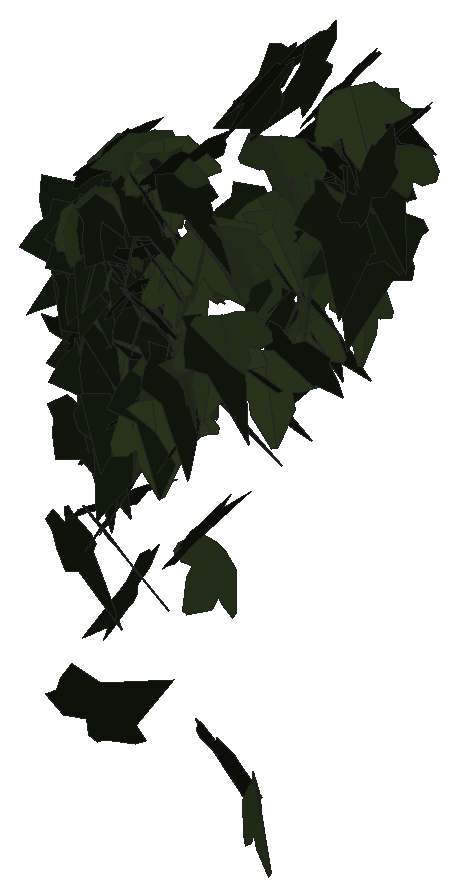
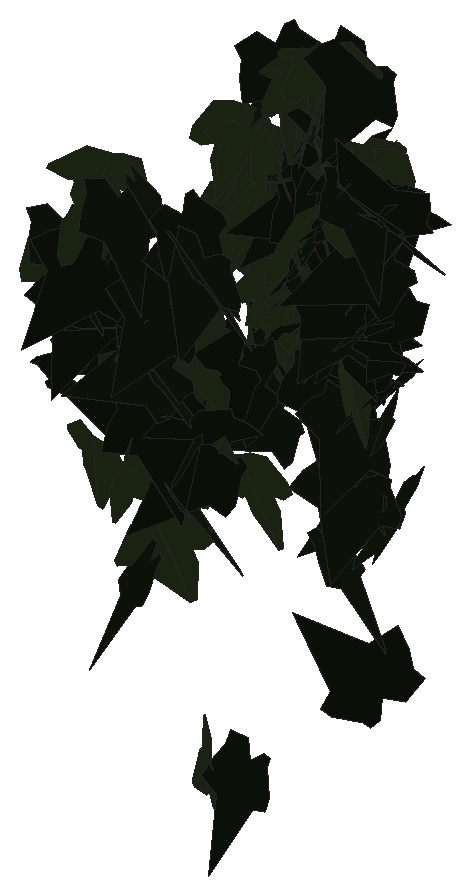
# SketchUp Ruby script. Lengths in inches.
U = 1.inch
M = Sketchup.active_model
def pt(a) = Geom::Point3d.new(a.map { |v| v * U })
def face(e, loops, mat)
  f = e.add_face(loops[0].map { |a| pt(a) })
  loops[1..].each { |l| e.add_face(l.map { |a| pt(a) }).erase! }
  f.material = f.back_material = mat if mat
  f
end
# faces: each face lists its corners as indices into pts; further lists are holes
def faces(e, pts, list, mat = nil) = list.each { |f| face(e, (f[0].is_a?(Array) ? f : [f]).map { |l| l.map { |i| pts[i] } }, mat) }
# xy, xz, yz: faces in a plane at the given z, y or x. An outline is a flat list of corners, or four numbers for a rectangle; further outlines are holes
def ring(l) = l.size == 4 ? [[l[0], l[1]], [l[2], l[1]], [l[2], l[3]], [l[0], l[3]]] : l.each_slice(2).to_a
def flat(e, list, mat, &to3) = list.each { |f| face(e, (f[0].is_a?(Array) ? f : [f]).map { |l| ring(l).map { |u, v| to3.(u, v) } }, mat) }
def xy(e, z, list, mat = nil) = flat(e, list, mat) { |x, y| [x, y, z] }
def xz(e, y, list, mat = nil) = flat(e, list, mat) { |x, z| [x, y, z] }
def yz(e, x, list, mat = nil) = flat(e, list, mat) { |y, z| [x, y, z] }
def lines(e, pts, list) = list.each { |a, b| e.add_line(pt(pts[a]), pt(pts[b])) }
# prism: a flat outline (further loops are holes) pulled along v
def prism(e, loops, v, mat = nil)
  f = face(e, loops, mat); d = Geom::Vector3d.new(v.map { |x| x * U })
  f.pushpull(f.normal.samedirection?(d) ? d.length : -d.length)
end
def box(e, o, s, mat = nil) = prism(e, [[o, [o[0] + s[0], o[1], o[2]], [o[0] + s[0], o[1] + s[1], o[2]], [o[0], o[1] + s[1], o[2]]]], [0, 0, s[2]], mat)
def at(x, y, z, deg = 0) = Geom::Transformation.translation(pt([x, y, z])) * Geom::Transformation.rotation(ORIGIN, Z_AXIS, deg.degrees)
def axes(o, x, y, z) = Geom::Transformation.new([*x, 0, *y, 0, *z, 0, *pt(o).to_a, 1])
def part(name) = M.definitions.add(name)
# library, detail: a bought-in or finely detailed component or shape, given as its bounding box
def library(name, o, s) = part(name).tap { |d| box(d.entities, o, s) }
def detail(e, o, s) = box(e.add_group.entities, o, s)
def put(e, d, t, mat = nil) = e.add_instance(d, t).tap { |i| i.material = mat if mat }
def group(e, t, mat = nil) = e.add_group.tap { |g| g.transformation = t; g.material = mat if mat }.entities
root = M.entities
M.materials.add("efeu1").color = [18, 25, 13]
M.materials.add("efeu2").color = [43, 57, 29]
c1 = part("ivyleaf_10")
p = [[0,0.5,-0.03],[-0.0625,2.02,-0.43],[-0.19,2.01,-0.46],[-0.54,1.05,-0.29],[-0.52,0.625,-0.18],[-0.83,0.76,-0.28],
  [-1.16,0.64,-0.33],[-1.15,0.33,-0.24],[-0.77,-0.39,0.02],[-0.3,-0.51,0.16],[0.04,-0.48,0.23],[-0.02,2.01,-0.4375],
  [-0.06,2.01,-0.43],[0.04,-0.49,0.23],[0.67,-0.49,0.14],[1.38,0.36,-0.2],[1.375,0.51,-0.24],[0.81,0.65,-0.19],
  [0.62,0.59,-0.15],[0.6,1.09,-0.28],[0.5,1.23,-0.31]]
faces(c1.entities,p,[[0,1,2,3,4,5,6,7,8,9,10],[11,12,0,13,14,15,16,17,18,19,20]],"efeu2")
c2 = part("ivyleaf_9")
p = [[1.54,2.16,1.25],[1.36,2.04,1.19],[-0.21,0.99,0.68],[-0.71,1.11,0.82],[-0.85,0.86,0.67],[-0.8,0.17,0.21],
  [-0.9,-0.01,0.1],[-0.67,-0.16,-0.02],[-0.08,-0.08,-0.05],[-0.03,-0.6,-0.4],[0.65,-0.88,-0.66],[0.83,-0.6,-0.49],
  [1.29,-0.42,-0.43],[1.8125,-0.07,-0.26],[1.21,0.44,0.15]]
faces(c2.entities,p,[[0,1,2,3,4,5,6,7,8,9,10,11,12,13,14]],"efeu1")
put(root,c1,axes([39.47,223.52,229.69],[0.36244,0.33716,0.07041],[0.0592,0.0397,-0.49489],[-0.33931,0.36708,-0.01114]))
put(root,c2,axes([39.32,223.59,231.17],[0.38837,-0.23519,0.20943],[0.19857,-0.0752,-0.45268],[0.24442,0.43478,0.03499]))
put(root,c2,axes([38.03,223.58,227.58],[0.35014,-0.34784,-0.08008],[-0.05711,0.05613,-0.49355],[0.35234,0.35477,-0.00042]))
put(root,c2,axes([38.21,223.69,231.0625],[0.23258,-0.43888,-0.05735],[-0.02686,0.05067,-0.4967],[0.4418,0.23413,0]))
put(root,c1,axes([39.18,223.65,233.53],[-0.2948,-0.40301,0.02593],[0.03422,-0.05692,-0.49557],[0.40239,-0.29042,0.06114]))
put(root,c2,axes([39.6,223.875,230.27],[0.11713,-0.47634,0.09688],[0.00471,-0.09853,-0.49017],[0.48606,0.11574,-0.01859]))
put(root,c2,axes([38.58,223.86,232.06],[-0.44079,-0.2001,-0.12514],[0.14056,-0.00962,-0.47974],[0.18959,-0.45811,0.06473]))
put(root,c2,axes([39.15,223.65,232.86],[0.30697,-0.38452,-0.08898],[-0.01554,0.10087,-0.48947],[0.39437,0.30327,0.04997]))
put(root,c2,axes([38.5625,223.8125,231.8],[-0.49937,0.02247,0.01106],[-0.01378,-0.06207,-0.49594],[-0.02091,-0.49562,0.06261]))
put(root,c1,axes([38.27,223.76,231.27],[0.29788,-0.38819,0.10286],[0.09191,-0.05877,-0.48795],[0.39092,0.30961,0.03635]))
put(root,c2,axes([38.2,223.72,229.26],[0.18322,-0.44715,-0.12841],[0.00533,0.14001,-0.47997],[0.46519,0.17451,0.05607]))
put(root,c1,axes([38.5,223.56,232.34],[0.37768,0.3074,0.11343],[0.02118,0.14983,-0.47655],[-0.32697,0.36477,0.10016]))
put(root,c2,axes([40.25,223.8125,231.06],[0.18899,-0.46289,-0.00354],[0.0162,0.01044,-0.49963],[0.46262,0.18873,0.01894]))
put(root,c2,axes([38.83,223.3,233.43],[0.13729,0.44226,0.18857],[0.0417,0.18441,-0.46288],[-0.47897,0.14282,0.01375]))
put(root,c2,axes([39.18,223.55,233.13],[0.44036,-0.1515,-0.18201],[-0.16409,0.08189,-0.46516],[0.17075,0.46941,0.02241]))
put(root,c1,axes([38.72,223.5625,231.48],[0.23486,-0.02081,0.44091],[0.40448,0.21012,-0.20554],[-0.17674,0.45323,0.11553]))
put(root,c1,axes([38.45,223.4375,232.35],[0.0695,0.43151,0.24284],[-0.08729,0.25206,-0.4229],[-0.48739,0.01639,0.11036]))
put(root,c2,axes([38.5,223.94,231.95],[-0.23311,-0.44222,-0.01025],[0.00224,0.0104,-0.49989],[0.44233,-0.2331,-0.00287]))
put(root,c2,axes([38.14,223.9,231.82],[-0.27892,-0.40327,-0.09788],[0.05985,0.07761,-0.4903],[0.41064,-0.28522,0.00498]))
put(root,c2,axes([38.33,223.66,224.9],[-0.00661,-0.09334,0.49117],[0.4885,-0.10574,-0.01352],[0.10639,0.47969,0.09259]))
put(root,c2,axes([38.99,223.77,231.15],[0.35335,-0.29827,0.19021],[0.1706,-0.09184,-0.46094],[0.30991,0.39064,0.03686]))
put(root,c1,axes([39.45,223.64,233.35],[-0.45934,-0.18071,-0.07968],[0.07468,0.02782,-0.49361],[0.18283,-0.46537,0.00143]))
put(root,c1,axes([38.98,223.92,232.48],[0.27341,-0.34521,0.23681],[0.14332,-0.18857,-0.44034],[0.39333,0.30867,-0.00417]))
put(root,c2,axes([38.51,223.8,232.26],[0.19981,-0.44967,-0.0887],[0.00539,0.09906,-0.49006],[0.45831,0.19488,0.04443]))
put(root,c2,axes([38.85,223.96,229.38],[-0.35138,-0.34494,-0.08687],[0.08765,0.03439,-0.49106],[0.34474,-0.36033,0.0363]))
put(root,c1,axes([39.17,223.77,232.15],[0.49484,-0.0273,0.06622],[0.06749,0.02308,-0.49489],[0.02396,0.49872,0.02653]))
put(root,c2,axes([38.89,223.91,232.4],[-0.37451,-0.23113,-0.23733],[0.22632,0.08306,-0.43804],[0.24191,-0.43552,0.0424]))
put(root,c2,axes([39.34,223.96,229.9375],[-0.07078,-0.49406,-0.02991],[0.00104,0.03007,-0.49909],[0.49496,-0.07071,-0.00323]))
put(root,c2,axes([39.65,223.82,233.21],[0.28258,-0.41215,-0.01663],[0.03246,0.04231,-0.49715],[0.41121,0.27989,0.05067]))
put(root,c2,axes([38.42,223.6875,227.75],[0.46646,-0.17963,-0.01195],[-0.01192,0.0023,-0.49985],[0.17963,0.46661,-0.00214]))
put(root,c2,axes([38.68,223.71,232.43],[0.15107,-0.39167,-0.27161],[-0.0986,0.25308,-0.4198],[0.46632,0.18039,-0.00078]))
put(root,c1,axes([39.89,223.84,232.07],[0.3598,-0.34718,0.00215],[0.00027,-0.00281,-0.49999],[0.34719,0.3598,-0.00183]))
put(root,c2,axes([38.35,223.9,231.875],[-0.0723,-0.47347,-0.14353],[0.00913,0.14376,-0.4788],[0.49466,-0.07186,-0.01215]))
put(root,c1,axes([40.45,223.76,231.27],[-0.36318,-0.34045,-0.04681],[0.07627,-0.01344,-0.49397],[0.33509,-0.36594,0.06169]))
put(root,c2,axes([38.15,224.06,228.54],[0.13393,-0.37777,0.29892],[0.09638,-0.28297,-0.4008],[0.47199,0.16498,-0.00297]))
put(root,c1,axes([39.13,223.76,231.29],[0.27709,-0.40303,-0.10386],[-0.04081,0.09786,-0.48863],[0.41419,0.27927,0.02133]))
put(root,c2,axes([38.94,223.74,228.46],[-0.30201,0.3759,-0.13226],[0.08643,-0.10021,-0.48217],[-0.389,-0.3141,-0.00445]))
put(root,c1,axes([39.27,223.72,233.02],[-0.28029,0.41238,-0.0371],[0.02268,-0.02945,-0.49862],[-0.41343,-0.2812,-0.00219]))
put(root,c1,axes([40.27,223.8125,230.97],[0.2864,0.4005,-0.08702],[-0.07084,-0.05618,-0.49176],[-0.40368,0.29401,0.02456]))
put(root,c2,axes([40.13,223.36,228.18],[0.18048,0.24838,0.39463],[0.09101,0.39626,-0.29103],[-0.45732,0.17688,0.09783]))
put(root,c1,axes([39.47,223.76,233.41],[0.30361,0.39596,0.03225],[0.02571,0.02093,-0.4989],[-0.39643,0.3046,-0.00765]))
put(root,c2,axes([39.84,223.77,233.59],[-0.12389,0.43002,-0.22301],[-0.00572,-0.23147,-0.44316],[-0.48438,-0.10725,0.06227]))
put(root,c1,axes([39.03,223.94,229.62],[-0.09984,0.42008,-0.25213],[-0.01238,-0.25939,-0.42728],[-0.48977,-0.07907,0.0622]))
put(root,c2,axes([38.49,224,230.02],[-0.2371,-0.42236,-0.12409],[0.0636,0.1066,-0.48435],[0.43559,-0.24546,0.00318]))
put(root,c1,axes([39.44,223.8,233.26],[-0.20706,-0.44492,-0.09578],[0.03838,0.08778,-0.49074],[0.45349,-0.21058,-0.0022]))
put(root,c2,axes([37.94,223.83,230.14],[0.25685,-0.14134,0.40503],[0.39799,-0.09769,-0.28647],[0.16011,0.46955,0.06232]))
put(root,c2,axes([39.1,224,231.02],[0.10467,-0.48677,-0.04587],[-0.00257,0.04636,-0.49784],[0.48892,0.10445,0.0072]))
put(root,c2,axes([39.27,223.72,231.59],[-0.05742,0.4833,-0.11457],[0.02731,-0.11208,-0.48651],[-0.49594,-0.06213,-0.01353]))
put(root,c2,axes([38.72,223.95,232.13],[0.23224,-0.43957,-0.05329],[0.0015,0.06095,-0.49627],[0.44279,0.23035,0.02963]))
put(root,c1,axes([39.86,223.84,230.68],[-0.48871,0.09336,-0.04944],[0.05001,-0.00164,-0.49749],[-0.09305,-0.4912,-0.00774]))
put(root,c1,axes([39.77,223.86,230.5],[-0.19734,0.45814,-0.03408],[-0.00458,-0.03905,-0.49845],[-0.45939,-0.19641,0.01961]))
put(root,c2,axes([39.87,223.75,229.64],[-0.24724,0.43166,0.05037],[-0.02029,0.04642,-0.49743],[-0.43412,-0.24801,-0.00544]))
put(root,c1,axes([38.95,223.98,231.625],[0.18918,0.44255,-0.13552],[-0.08262,-0.11176,-0.4803],[-0.4554,0.20411,0.03084]))
put(root,c2,axes([38.97,223.63,231.65],[0.34442,0.14416,0.33255],[0.29461,0.15589,-0.3727],[-0.21113,0.45268,0.02244]))
put(root,c2,axes([38.875,223.88,226.88],[-0.33198,0.37281,-0.02829],[0.01925,-0.02074,-0.4992],[-0.37338,-0.33254,-0.00058]))
put(root,c2,axes([39.09,223.77,231.96],[0.41366,0.01833,-0.28027],[-0.28079,0.03879,-0.41189],[0.00665,0.49816,0.04239]))
put(root,c1,axes([38.32,223.97,231.64],[-0.00115,-0.49749,0.05002],[-0.00117,0.05002,0.49749],[-0.5,0.00103,-0.00128]))
put(root,c1,axes([39.6875,223.86,230.39],[-0.30373,-0.34577,-0.19543],[0.13739,0.13937,-0.46011],[0.37265,-0.3332,0.01035]))
put(root,c1,axes([39.3125,223.99,229.61],[0.44393,0.22931,0.01841],[0.01929,0.00277,-0.49962],[-0.22924,0.44431,-0.00639]))
put(root,c1,axes([39.65,223.95,231.66],[0.31466,0.38699,-0.03511],[-0.06041,0.00409,-0.49632],[-0.38385,0.31658,0.04932]))
put(root,c1,axes([39.41,223.9,230.18],[-0.44097,0.14775,0.18361],[-0.19097,0.00426,-0.46208],[-0.13811,-0.47765,0.05267]))
put(root,c1,axes([39.41,223.96,230.25],[-0.35636,-0.34181,-0.07856],[0.09583,0.01284,-0.49056],[0.33738,-0.36469,0.05636]))
put(root,c2,axes([38.31,224.2,230.04],[-0.35844,-0.31216,-0.15516],[0.14766,0.06564,-0.47317],[0.31578,-0.38503,0.04513]))
put(root,c1,axes([38.74,224.02,230.78],[0.3233,0.37082,-0.08926],[-0.08072,-0.04784,-0.49112],[-0.37277,0.33197,0.02893]))
put(root,c2,axes([38.08,223.875,231.82],[-0.35763,0.04846,0.34606],[0.34276,-0.04768,0.36089],[0.06798,0.49536,0.00088]))
put(root,c1,axes([40.3,223.96,232.4375],[-0.49051,-0.08691,-0.04298],[0.04153,0.01198,-0.49813],[0.08762,-0.49224,-0.00453]))
put(root,c1,axes([39.18,224.04,231.11],[-0.19915,-0.45451,-0.06135],[0.13786,0.00447,-0.4806],[0.43742,-0.20834,0.12354]))
put(root,c2,axes([39.1,223.78,231.91],[0.47563,0.15114,0.03055],[0.01391,0.05661,-0.49659],[-0.15357,0.47323,0.04964]))
put(root,c1,axes([40.07,224.01,227.59],[0.44016,-0.1022,-0.21404],[-0.19101,0.11476,-0.4476],[0.14061,0.4758,0.06199]))
put(root,c2,axes([38.37,224.1,230.125],[0.16226,-0.44862,-0.1497],[-0.00896,0.15532,-0.47518],[0.47285,0.15689,0.04237]))
put(root,c1,axes([40.01,223.86,232.28],[0.21528,0.34681,0.28875],[0.11126,0.26926,-0.40635],[-0.43735,0.23921,0.03876]))
put(root,c1,axes([40.12,224.03,232.25],[-0.47295,0.07346,0.14465],[-0.14666,-0.00303,-0.478],[-0.06935,-0.49457,0.02441]))
put(root,c2,axes([38.42,223.94,232.14],[-0.11889,0.48566,-0.00072],[-0.00196,-0.00122,-0.49999],[-0.48565,-0.11889,0.0022]))
put(root,c1,axes([39.27,224.15,230.99],[0.31954,-0.368,-0.11168],[-0.04455,0.10879,-0.48598],[0.38198,0.32054,0.03674]))
put(root,c1,axes([38.28,224.27,229.78],[0.15643,-0.47487,-0.0047],[-0.0027,0.00406,-0.49998],[0.47489,0.15645,-0.0013]))
put(root,c2,axes([38.8125,223.98,229.35],[0.03369,0.49886,-0.00194],[0.00026,-0.00196,-0.5],[-0.49886,0.03369,-0.00039]))
put(root,c2,axes([37.99,223.9,231.29],[0.39857,0.1536,0.25991],[0.19827,0.19144,-0.41718],[-0.22767,0.43561,0.0917]))
put(root,c2,axes([38.59,224.29,230.68],[-0.16226,0.37919,-0.28264],[0.11779,-0.257,-0.41241],[-0.45804,-0.20042,-0.00593]))
put(root,c2,axes([38.4375,223.94,227.98],[0.18725,0.45827,0.07018],[-0.10692,0.11634,-0.47438],[-0.45112,0.16265,0.14156]))
put(root,c2,axes([38.39,224.03,228.89],[0.11654,0.44873,0.18725],[-0.00314,0.19325,-0.46113],[-0.48622,0.1063,0.04786]))
put(root,c2,axes([38.61,224.07,230.45],[0.13044,0.38696,0.28852],[-0.00744,0.30045,-0.39959],[-0.48263,0.09996,0.08414]))
put(root,c1,axes([40.05,224.83,223.75],[0.22925,-0.18036,0.4061],[0.38633,-0.14486,-0.28243],[0.21953,0.44327,0.07294]))
put(root,c2,axes([39.16,224.94,229.53],[0.46862,-0.16869,0.04399],[0.04328,-0.00966,-0.49803],[0.16888,0.47058,0.00555]))
put(root,c1,axes([40.08,225.02,229.96],[0.41569,0.25761,0.10411],[0.07812,0.07143,-0.48867],[-0.26665,0.42253,0.01914]))
put(root,c2,axes([40.53,225.06,230.47],[0.31333,0.1671,-0.35199],[-0.31422,-0.15873,-0.35506],[-0.23041,0.44371,0.00555]))
put(root,c2,axes([39.5,225.07,229.75],[0.49894,0.02587,0.01963],[0.01942,0.00472,-0.4996],[-0.02604,0.49931,0.0037]))
put(root,c2,axes([39.27,225.09,224.18],[0.4242,0.02656,-0.26334],[-0.26414,0.01084,-0.42439],[-0.01683,0.49918,0.02322]))
put(root,c2,axes([40.75,226.37,232.22],[-0.08275,0.24388,0.42857],[-0.24275,0.35811,-0.25066],[-0.42921,-0.24955,0.05914]))
put(root,c2,axes([39.625,226.39,230.59],[-0.02964,0.4632,0.18591],[-0.04946,0.1826,-0.46283],[-0.49666,-0.04583,0.03499]))
put(root,c1,axes([40.18,226.74,233.11],[0.35416,0.32651,0.13402],[0.08745,0.10276,-0.48145],[-0.34194,0.36446,0.01568]))
put(root,c1,axes([38.83,226.86,231.95],[-0.48219,-0.06452,-0.11545],[0.11568,0.00581,-0.4864],[0.06411,-0.49579,0.00933]))
put(root,c1,axes([38.52,226.99,230.8],[0.38012,0.09073,0.31189],[0.3021,0.07765,-0.39078],[-0.11934,0.48553,0.00421]))
put(root,c2,axes([38.68,227.07,233.02],[-0.23066,0.38636,-0.21799],[0.06858,-0.21169,-0.44775],[-0.43828,-0.23646,0.04466]))
put(root,c1,axes([38.84,227.25,230.5625],[-0.25608,-0.26061,0.34133],[-0.19044,-0.28728,-0.36221],[0.38491,-0.31552,0.04787]))
put(root,c2,axes([40.18,227.22,232.04],[0.18562,-0.46277,0.03723],[0.01671,-0.03341,-0.4986],[0.46397,0.18634,0.00306]))
put(root,c2,axes([39.61,227.34,231.13],[-0.02666,-0.49707,0.04699],[-0.00802,-0.04663,-0.49776],[0.49922,-0.0273,-0.00548]))
put(root,c2,axes([39.33,227.14,233.28],[-0.42234,0.24732,-0.10228],[0.07704,-0.07066,-0.48895],[-0.25631,-0.42877,0.02158]))
put(root,c2,axes([39.57,226.94,232.1],[0.49609,-0.01215,-0.0612],[-0.06106,0.00647,-0.49622],[0.01285,0.49981,0.00494]))
put(root,c2,axes([39.9,226.9375,232.49],[0.35326,-0.13864,-0.32555],[-0.29045,0.14914,-0.37868],[0.2021,0.45666,0.02484]))
put(root,c1,axes([39.36,227.24,231.21],[-0.40713,-0.15969,0.24238],[-0.19379,-0.1613,-0.43178],[0.21609,-0.44551,0.06944]))
put(root,c1,axes([38.92,227.34,230.17],[0.37041,-0.25914,0.21364],[0.19519,-0.09273,-0.45089],[0.27331,0.41743,0.03247]))
put(root,c1,axes([38.35,227.2,230.11],[0.49889,-0.03238,0.0076],[0.01252,0.07699,-0.49388],[0.03081,0.49298,0.07763]))
put(root,c2,axes([38.56,227.16,232.64],[-0.39006,0.30751,0.05732],[-0.04055,0.04114,-0.49665],[-0.31017,-0.3921,-0.00716]))
put(root,c1,axes([40.42,227.32,232.18],[-0.35553,-0.34009,0.08911],[-0.03473,-0.09213,-0.49021],[0.34985,-0.35476,0.04188]))
put(root,c1,axes([39.88,227.43,232.74],[-0.17413,-0.45991,0.09036],[-0.01042,-0.09258,-0.49124],[0.46858,-0.17296,0.02266]))
put(root,c2,axes([38.42,227.27,230.18],[0.43784,-0.23049,-0.07191],[-0.04809,0.06269,-0.49372],[0.23661,0.43926,0.03273]))
put(root,c2,axes([38.19,227.56,230.5],[-0.29382,-0.38326,-0.12956],[0.08268,0.09986,-0.4829],[0.39602,-0.30519,0.0047]))
put(root,c2,axes([38.63,227.37,229.45],[-0.40643,0.28932,0.03328],[-0.03896,0.0026,-0.49847],[-0.28861,-0.40779,0.02043]))
put(root,c2,axes([38.71,227.55,230.99],[-0.45405,0.12159,-0.17045],[0.14313,-0.11683,-0.46461],[-0.15281,-0.47071,0.07128]))
put(root,c1,axes([39.72,227.35,232.06],[-0.49856,-0.0055,-0.0375],[0.03744,0.00548,-0.49857],[0.00589,-0.49994,-0.00505]))
put(root,c2,axes([39.58,227.24,233.02],[-0.11985,0.48533,-0.00964],[-0.00168,-0.01034,-0.49989],[-0.48542,-0.11979,0.00411]))
put(root,c2,axes([40.34,227.36,232.48],[-0.15408,0.47273,-0.05273],[-0.03874,-0.06771,-0.49388],[-0.47409,-0.14811,0.05749]))
put(root,c2,axes([40,227.82,231.01],[-0.36682,-0.25859,0.2204],[-0.18743,-0.11652,-0.44866],[0.2834,-0.41177,-0.01145]))
put(root,c1,axes([38.94,227.36,231.46],[-0.06065,0.48387,0.1104],[-0.02002,0.10874,-0.48762],[-0.4959,-0.06357,0.00618]))
put(root,c2,axes([38.3125,227.18,232.6],[0.08221,0.47138,0.14507],[-0.0323,0.1519,-0.47527],[-0.49214,0.06877,0.05543]))
put(root,c2,axes([38.0625,227.26,229.96],[0.42011,0.24453,0.11709],[0.10145,0.05846,-0.4861],[-0.25142,0.43219,-0.0005]))
put(root,c2,axes([39.69,227.76,230.55],[-0.37494,-0.24598,-0.22116],[0.23042,0.04563,-0.44139],[0.23733,-0.43291,0.07914]))
put(root,c2,axes([38.7,227.47,230.48],[0.1543,0.40907,-0.24259],[-0.16895,-0.19126,-0.42997],[-0.44457,0.21466,0.07921]))
put(root,c1,axes([38.87,227.9,229.77],[0.02923,0.29142,-0.40524],[-0.12578,-0.38853,-0.28848],[-0.48304,0.1188,0.0506]))
put(root,c2,axes([38.81,227.26,231.82],[0.16052,0.42236,0.21411],[0.07592,0.2002,-0.45184],[-0.46741,0.17757,0.00014]))
put(root,c1,axes([38.53,227.68,228.875],[0.36064,0.30839,-0.15757],[-0.18915,-0.01516,-0.46259],[-0.2901,0.39327,0.10574]))
put(root,c1,axes([39.5,227.77,229.78],[0.47277,-0.10194,0.12687],[0.12539,-0.02032,-0.4836],[0.10375,0.48908,0.00635]))
put(root,c2,axes([38.71,227.38,231.04],[0.37082,0.12701,0.31042],[0.17681,0.31921,-0.34183],[-0.28501,0.36328,0.19183]))
put(root,c2,axes([39.68,227.54,231.85],[0.30074,0.39931,-0.01033],[-0.00583,-0.00853,-0.49989],[-0.3994,0.30079,-0.00048]))
put(root,c2,axes([39.68,227.53,232.27],[0.32327,0.35262,0.14546],[0.09832,0.1072,-0.47837],[-0.36855,0.33789,-0.00003]))
put(root,c2,axes([38.35,228.23,228.71],[0.38658,-0.08218,-0.30627],[-0.26555,0.18004,-0.3835],[0.17331,0.45916,0.09555]))
